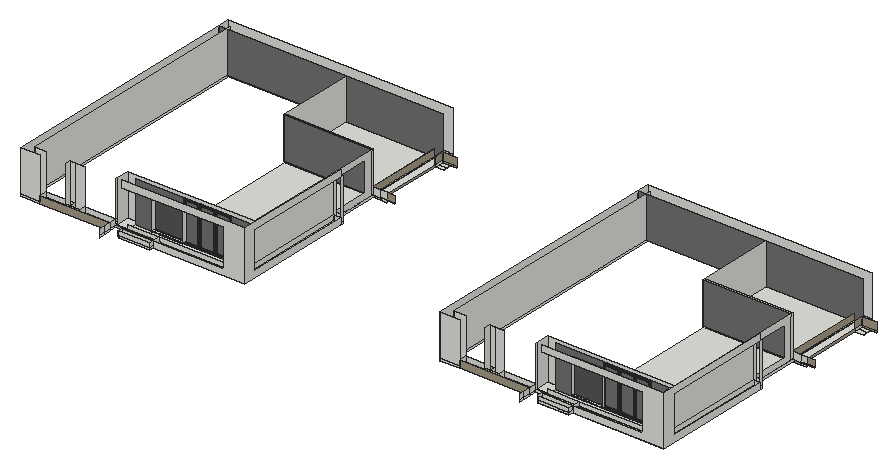
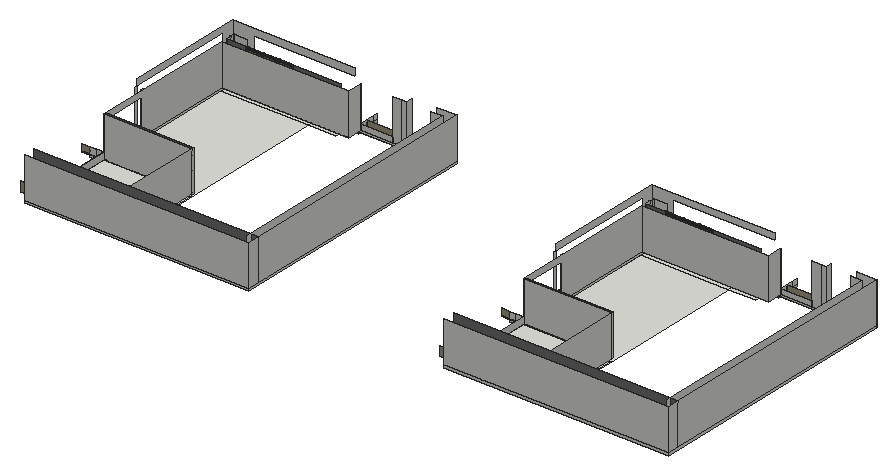
# SketchUp Ruby script. Lengths in inches.
U = 1.inch
M = Sketchup.active_model
def pt(a) = Geom::Point3d.new(a.map { |v| v * U })
def face(e, loops, mat)
  f = e.add_face(loops[0].map { |a| pt(a) })
  loops[1..].each { |l| e.add_face(l.map { |a| pt(a) }).erase! }
  f.material = f.back_material = mat if mat
  f
end
# faces: each face lists its corners as indices into pts; further lists are holes
def faces(e, pts, list, mat = nil) = list.each { |f| face(e, (f[0].is_a?(Array) ? f : [f]).map { |l| l.map { |i| pts[i] } }, mat) }
# xy, xz, yz: faces in a plane at the given z, y or x. An outline is a flat list of corners, or four numbers for a rectangle; further outlines are holes
def ring(l) = l.size == 4 ? [[l[0], l[1]], [l[2], l[1]], [l[2], l[3]], [l[0], l[3]]] : l.each_slice(2).to_a
def flat(e, list, mat, &to3) = list.each { |f| face(e, (f[0].is_a?(Array) ? f : [f]).map { |l| ring(l).map { |u, v| to3.(u, v) } }, mat) }
def xy(e, z, list, mat = nil) = flat(e, list, mat) { |x, y| [x, y, z] }
def xz(e, y, list, mat = nil) = flat(e, list, mat) { |x, z| [x, y, z] }
def yz(e, x, list, mat = nil) = flat(e, list, mat) { |y, z| [x, y, z] }
def lines(e, pts, list) = list.each { |a, b| e.add_line(pt(pts[a]), pt(pts[b])) }
# prism: a flat outline (further loops are holes) pulled along v
def prism(e, loops, v, mat = nil)
  f = face(e, loops, mat); d = Geom::Vector3d.new(v.map { |x| x * U })
  f.pushpull(f.normal.samedirection?(d) ? d.length : -d.length)
end
def box(e, o, s, mat = nil) = prism(e, [[o, [o[0] + s[0], o[1], o[2]], [o[0] + s[0], o[1] + s[1], o[2]], [o[0], o[1] + s[1], o[2]]]], [0, 0, s[2]], mat)
def at(x, y, z, deg = 0) = Geom::Transformation.translation(pt([x, y, z])) * Geom::Transformation.rotation(ORIGIN, Z_AXIS, deg.degrees)
def axes(o, x, y, z) = Geom::Transformation.new([*x, 0, *y, 0, *z, 0, *pt(o).to_a, 1])
def part(name) = M.definitions.add(name)
# library, detail: a bought-in or finely detailed component or shape, given as its bounding box
def library(name, o, s) = part(name).tap { |d| box(d.entities, o, s) }
def detail(e, o, s) = box(e.add_group.entities, o, s)
def put(e, d, t, mat = nil) = e.add_instance(d, t).tap { |i| i.material = mat if mat }
def group(e, t, mat = nil) = e.add_group.tap { |g| g.transformation = t; g.material = mat if mat }.entities
root = M.entities
M.materials.add("Wine2").color = [0, 0, 0]
M.materials["Wine2"].alpha = 0
M.materials.add("[0130_Gainsboro]").color = [39, 45, 50]
M.materials.add("[Color M05]").color = [114, 114, 114]
M.materials.add("[Color M06]").color = [86, 86, 86]
M.materials.add("[Concrete Tile]").color = [165, 155, 133]
M.materials.add("[Granite Brown]").color = [89, 59, 61]
c1 = part("Framed glazing panel")
xy(c1.entities,0,[[0,-0.98,43.07,0],[0,0,43.07,1.4]],"[0130_Gainsboro]")
xy(c1.entities,0.3,[[0.3,-1.43,42.77,-0.98]],"[0130_Gainsboro]")
xy(c1.entities,2.95,[[2.95,-1.43,40.12,-0.63],[2.95,-0.63,40.12,0],[2.95,0,40.12,0.64],[2.95,0.64,40.12,1.4]],"[0130_Gainsboro]")
xy(c1.entities,3.54,[[3.54,-0.63,39.53,0],[3.54,0,39.53,0.64]],"[0130_Gainsboro]")
xy(c1.entities,111.8125,[[3.54,-0.63,39.53,0],[3.54,0,39.53,0.64]],"[0130_Gainsboro]")
xy(c1.entities,112.4,[[2.95,-1.43,40.12,-0.63],[2.95,-0.63,40.12,0],[2.95,0,40.12,0.64],[2.95,0.64,40.12,1.4]],"[0130_Gainsboro]")
xy(c1.entities,115.05,[[0.3,-1.43,42.77,-0.98]],"[0130_Gainsboro]")
xy(c1.entities,115.35,[[0,-0.98,43.07,0],[0,0,43.07,1.4]],"[0130_Gainsboro]")
xz(c1.entities,-1.43,[[[0.3,0.3,42.77,115.05],[2.95,2.95,40.12,112.4]]],"[0130_Gainsboro]")
xz(c1.entities,-0.98,[[[0,0,43.07,115.35],[0.3,0.3,42.77,115.05]]],"[0130_Gainsboro]")
xz(c1.entities,-0.63,[[[2.95,2.95,40.12,112.4],[3.54,3.54,39.53,111.8125]]],"[0130_Gainsboro]")
xz(c1.entities,0,[[3.54,3.54,39.53,111.8125]],"Wine2")
xz(c1.entities,0,[[[0,0,43.07,115.35],[2.95,2.95,40.12,112.4]],[[2.95,2.95,40.12,112.4],[3.54,3.54,39.53,111.8125]]],"[0130_Gainsboro]")
xz(c1.entities,0.64,[[[2.95,2.95,40.12,112.4],[3.54,3.54,39.53,111.8125]]],"[0130_Gainsboro]")
xz(c1.entities,1.4,[[[0,0,43.07,115.35],[2.95,2.95,40.12,112.4]]],"[0130_Gainsboro]")
yz(c1.entities,0,[[-0.98,0,0,115.35],[0,0,1.4,115.35]],"[0130_Gainsboro]")
yz(c1.entities,0.3,[[-1.43,0.3,-0.98,115.05]],"[0130_Gainsboro]")
yz(c1.entities,2.95,[[-1.43,2.95,-0.63,112.4],[-0.63,2.95,0,112.4],[0,2.95,0.64,112.4],[0.64,2.95,1.4,112.4]],"[0130_Gainsboro]")
yz(c1.entities,3.54,[[-0.63,3.54,0,111.8125],[0,3.54,0.64,111.8125]],"[0130_Gainsboro]")
yz(c1.entities,39.53,[[-0.63,3.54,0,111.8125],[0,3.54,0.64,111.8125]],"[0130_Gainsboro]")
yz(c1.entities,40.12,[[-1.43,2.95,-0.63,112.4],[-0.63,2.95,0,112.4],[0,2.95,0.64,112.4],[0.64,2.95,1.4,112.4]],"[0130_Gainsboro]")
yz(c1.entities,42.77,[[-1.43,0.3,-0.98,115.05]],"[0130_Gainsboro]")
yz(c1.entities,43.07,[[-0.98,0,0,115.35],[0,0,1.4,115.35]],"[0130_Gainsboro]")
c2 = part("Glazed panel assembly")
put(c2.entities,c1,axes([90.57,1.43,0],[1.05148,0,0],[0,1,0],[0,0,1]))
put(c2.entities,c1,axes([0,1.43,0],[1.05148,0,0],[0,1,0],[0,0,1]))
put(c2.entities,c1,axes([45.29,1.43,0],[1.05148,0,0],[0,1,0],[0,0,1]))
xy(root,882,[[558.21,1786.97,648.68,1822.9375],[1776.4,1786.97,1866.87,1822.9375],[319.53,1799.9375,319.53,1822.9375,403.03,1822.9375,403.03,1806.5625,446.15,1806.5625,446.15,1822.9375,523.04,1822.9375,523.04,1799.9375],[648.68,1799.9375,648.68,1822.9375,890.875,1822.9375,890.875,1842.5,913.875,1842.5,913.875,1799.9375],[1537.72,1799.9375,1537.72,1822.9375,1621.22,1822.9375,1621.22,1806.5625,1664.33,1806.5625,1664.33,1822.9375,1741.23,1822.9375,1741.23,1799.9375],
  [1866.87,1799.9375,1866.87,1822.9375,2109.0625,1822.9375,2109.0625,1842.5,2132.0625,1842.5,2132.0625,1799.9375],[431.33,1806.5625,446.15,1822.9375],[1649.52,1806.5625,1664.33,1822.9375],[523.04,1822.9375,557.4,1822.9375,557.4,1826.625,557.88,1826.625,557.88,1830.25,523.04,1830.25],[648.68,1822.9375,890.875,1822.9375,890.875,1842.5,635.3125,1842.5,635.3125,1826.625,648.68,1826.625],
  [1741.23,1822.9375,1775.59,1822.9375,1775.59,1826.625,1776.07,1826.625,1776.07,1830.25,1741.23,1830.25],[1866.87,1822.9375,2109.0625,1822.9375,2109.0625,1842.5,1853.5,1842.5,1853.5,1826.625,1866.87,1826.625],[557.88,1826.625,635.3125,1830.25],[1776.07,1826.625,1853.5,1830.25],[557.88,1830.25,635.3125,1842.5],
  [1776.07,1830.25,1853.5,1842.5],[557.4,1842.5,635.3125,1869.5],[635.3125,1842.5,890.875,1869.5],[890.875,1842.5,891.6875,1869.5],[891.6875,1842.5,894.3125,2148.83],
  [894.3125,1842.5,913.875,2148.83],[1775.59,1842.5,1853.5,1869.5],[1853.5,1842.5,2109.0625,1869.5],[2109.0625,1842.5,2109.875,1869.5],[2109.875,1842.5,2112.5,2148.83],
  [2112.5,1842.5,2132.0625,2148.83],[635.3125,1869.5,890.875,2295.875],[1853.5,1869.5,2109.0625,2295.875],[894,2148.83,894.3125,2156.01],[894.3125,2148.83,913.875,2156.01],
  [2112.1875,2148.83,2112.5,2156.01],[2112.5,2148.83,2132.0625,2156.01],[635.3125,2295.875,637.0625,2518.89],[637.0625,2295.875,637.0625,2518.89,889.625,2518.89,889.625,2492.875,890.875,2492.875,890.875,2295.875],[1853.5,2295.875,1855.25,2518.89],
  [1855.25,2295.875,1855.25,2518.89,2107.8125,2518.89,2107.8125,2492.875,2109.0625,2492.875,2109.0625,2295.875],[889.625,2492.875,890.875,2518.89],[890.875,2492.875,912.625,2505.5625],[912.625,2492.875,913.875,2505.5625],[913.875,2492.875,938.375,2505.5625],
  [938.375,2492.875,938.5625,2518.89],[2107.8125,2492.875,2109.0625,2518.89],[2109.0625,2492.875,2130.8125,2505.5625],[2130.8125,2492.875,2132.0625,2505.5625],[2132.0625,2492.875,2156.5625,2505.5625],
  [2156.5625,2492.875,2156.75,2518.89],[890.875,2505.5625,912.625,2518.89],[912.625,2505.5625,913.875,2518.89],[913.875,2505.5625,938.375,2518.89],[2109.0625,2505.5625,2130.8125,2518.89],
  [2130.8125,2505.5625,2132.0625,2518.89],[2132.0625,2505.5625,2156.5625,2518.89],[635.3125,2518.89,890.875,2531.375],[1853.5,2518.89,2109.0625,2531.375]])
xy(root,882,[[890.875,2295.875,913.875,2492.875],[2109.0625,2295.875,2132.0625,2492.875]],"[Concrete Tile]")
xy(root,882,[[557.4,1822.9375,557.88,1826.625],[1775.59,1822.9375,1776.07,1826.625]],"[Granite Brown]")
xy(root,888,[[557.88,1786.97,558.21,1799.9375],[558.21,1786.97,647.87,1799.9375],[647.87,1786.97,648.68,1799.9375],[1776.07,1786.97,1776.4,1799.9375],[1776.4,1786.97,1866.06,1799.9375],
  [1866.06,1786.97,1866.87,1799.9375],[557.88,1799.9375,558.21,1822.9375],[558.21,1799.9375,647.87,1822.9375],[647.87,1799.9375,648.68,1822.9375],[1776.07,1799.9375,1776.4,1822.9375],
  [1776.4,1799.9375,1866.06,1822.9375],[1866.06,1799.9375,1866.87,1822.9375],[523.04,1822.9375,557.4,1826.625],[648.68,1822.9375,890.875,1826.625],[1741.23,1822.9375,1775.59,1826.625],
  [1866.87,1822.9375,2109.0625,1826.625],[523.04,1826.625,523.04,1865.75,557.4,1865.75,557.4,1850.9375,557.88,1850.9375,557.88,1826.625],[557.88,1826.625,890.875,1850.9375],[1741.23,1826.625,1741.23,1865.75,1775.59,1865.75,1775.59,1850.9375,1776.07,1850.9375,1776.07,1826.625],[1776.07,1826.625,2109.0625,1850.9375],
  [557.4,1850.9375,890.875,1865.75],[1775.59,1850.9375,2109.0625,1865.75],[894.3125,2148.83,913.875,2156.01],[2112.5,2148.83,2132.0625,2156.01],[635.3125,2290,890.875,2295.875],
  [1853.5,2290,2109.0625,2295.875],[890.875,2295.875,890.875,2517.14,912.625,2517.14,912.625,2492.875,913.875,2492.875,913.875,2295.875],[2109.0625,2295.875,2109.0625,2517.14,2130.8125,2517.14,2130.8125,2492.875,2132.0625,2492.875,2132.0625,2295.875],[912.625,2492.875,913.875,2517.14],[2130.8125,2492.875,2132.0625,2517.14],
  [890.875,2517.14,912.625,2518.64],[912.625,2517.14,913.875,2518.64],[2109.0625,2517.14,2130.8125,2518.64],[2130.8125,2517.14,2132.0625,2518.64],[890.875,2518.64,912.625,2518.89],
  [912.625,2518.64,913.875,2518.89],[2109.0625,2518.64,2130.8125,2518.89],[2130.8125,2518.64,2132.0625,2518.89],[285.875,2519.125,890.875,2531.375],[1504.0625,2519.125,2109.0625,2531.375]])
xy(root,888,[[557.4,1786.97,557.88,1799.9375],[1775.59,1786.97,1776.07,1799.9375],[557.4,1822.9375,557.88,1826.625],[1775.59,1822.9375,1776.07,1826.625]],"[Granite Brown]")
xy(root,889.75,[[635.3125,2295.875,889.625,2517.14],[889.625,2295.875,890.875,2517.14],[1853.5,2295.875,2107.8125,2517.14],[2107.8125,2295.875,2109.0625,2517.14]])
xy(root,895.375,[[632.49,1842.5,648.79,1850.9375],[648.79,1842.5,650.48,1850.9375],[650.48,1842.5,701.59,1850.9375],[1850.67,1842.5,1866.98,1850.9375],[1866.98,1842.5,1868.66,1850.9375],
  [1868.66,1842.5,1919.77,1850.9375]])
xy(root,895.6875,[[611.65,1842.5,632.49,1850.9375],[1829.84,1842.5,1850.67,1850.9375]])
xz(root,1786.97,[[558.21,882,648.68,888],[1776.4,882,1866.87,888],[557.88,888,647.87,900.6875],[1776.07,888,1866.06,900.6875]])
xz(root,1786.97,[[557.4,888,557.88,900.6875],[1775.59,888,1776.07,900.6875]],"[Granite Brown]")
xz(root,1799.9375,[[262.875,882,319.53,888],[648.68,882,913.875,882,913.875,1026.6875,557.88,1026.6875,557.88,1008,852.99,1008,852.99,900.6875,647.87,900.6875,647.87,888,648.68,888],[1481.0625,882,1537.72,888],[1866.87,882,2132.0625,882,2132.0625,1026.6875,1776.07,1026.6875,1776.07,1008,2071.18,1008,2071.18,900.6875,1866.06,900.6875,1866.06,888,1866.87,888],[262.875,888,319.53,1008],
  [557.4,888,647.87,900.6875],[1481.0625,888,1537.72,1008],[1775.59,888,1866.06,900.6875]])
xz(root,1799.9375,[[319.53,882,523.04,903.4375],[1537.72,882,1741.23,903.4375]],"[Concrete Tile]")
xz(root,1806.5625,[[403.0625,888,403.0625,903.4375,388.33,903.51,388.25,888.07],[403.0625,888,403.14,903.4375,403.0625,903.4375],[403.0625,888,431.33,888,431.33,903.4375,403.14,903.4375],[1621.25,888,1621.25,903.4375,1606.52,903.51,1606.4375,888.07],[1621.25,888,1621.33,903.4375,1621.25,903.4375],
  [1621.25,888,1649.52,888,1649.52,903.4375,1621.33,903.4375]])
xz(root,1822.9375,[[285.875,882,557.4,888],[558.21,882,648.68,888],[648.68,882,890.875,888],[1504.0625,882,1775.59,888],[1776.4,882,1866.87,888],
  [1866.87,882,2109.0625,888],[285.875,888,319.53,1008],[319.53,888,403.0625,888,388.25,888.07,388.33,903.4375,319.53,903.4375],[403.0625,888,388.25,888.07,388.33,903.4375,403.0625,903.4375],[403.0625,888,403.66,1008,388.85,1008,388.33,903.4375,403.0625,903.4375],
  [403.0625,888,403.66,1008,431.33,1008,431.33,888],[431.33,888,523.04,903.4375],[557.88,888,647.87,900.6875],[647.87,888,647.87,900.6875,852.99,900.6875,852.99,1008,890.875,1008,890.875,888],[1504.0625,888,1537.72,1008],
  [1537.72,888,1621.25,888,1606.4375,888.07,1606.52,903.4375,1537.72,903.4375],[1621.25,888,1606.4375,888.07,1606.52,903.4375,1621.25,903.4375],[1621.25,888,1621.85,1008,1607.04,1008,1606.52,903.4375,1621.25,903.4375],[1621.25,888,1621.85,1008,1649.52,1008,1649.52,888],[1649.52,888,1741.23,903.4375],
  [1776.07,888,1866.06,900.6875],[1866.06,888,1866.06,900.6875,2071.18,900.6875,2071.18,1008,2109.0625,1008,2109.0625,888]])
xz(root,1822.9375,[[557.4,882,557.88,888],[1775.59,882,1776.07,888]],"[Granite Brown]")
xz(root,1826.625,[[557.4,882,648.68,888],[1775.59,882,1866.87,888]])
xz(root,1835.1875,[[890.875,888,894.3125,1008],[2109.0625,888,2112.5,1008]])
xz(root,1842.5,[[632.49,893.4375,701.59,893.4375,701.59,895.375,632.49,895.375,632.49,895.6875,611.65,895.6875,611.65,893.75,632.49,893.75],[1850.67,893.4375,1919.77,893.4375,1919.77,895.375,1850.67,895.375,1850.67,895.6875,1829.84,895.6875,1829.84,893.75,1850.67,893.75]])
xz(root,1850.9375,[[[557.88,888,890.875,888,890.875,1008,557.88,1008,557.88,986.96,557.4,986.96,557.4,934.68,557.88,934.68],[632.49,895.375,632.49,895.6875,611.65,895.6875,611.65,991.5625,701.59,991.5625,701.59,895.375]],[[1776.07,888,2109.0625,888,2109.0625,1008,1776.07,1008,1776.07,986.96,1775.59,986.96,1775.59,934.68,1776.07,934.68],[1850.67,895.375,1850.67,895.6875,1829.84,895.6875,1829.84,991.5625,1919.77,991.5625,1919.77,895.375]]],"[Color M05]")
xz(root,1850.9375,[[632.49,895.375,701.59,895.375,701.59,991.5625,611.65,991.5625,611.65,895.6875,632.49,895.6875],[1850.67,895.375,1919.77,895.375,1919.77,991.5625,1829.84,991.5625,1829.84,895.6875,1850.67,895.6875]],"[Color M06]")
xz(root,1865.75,[[523.04,888,890.875,1008],[1741.23,888,2109.0625,1008]])
xz(root,2148.83,[[894.3125,882,913.875,888],[2112.5,882,2132.0625,888],[894.3125,888,913.875,900.6875],[2112.5,888,2132.0625,900.6875]])
xz(root,2156.01,[[894.3125,882,913.875,888],[2112.5,882,2132.0625,888],[894.3125,888,913.875,905.36],[2112.5,888,2132.0625,905.36]])
xz(root,2290,[[635.3125,888,890.875,1008],[1853.5,888,2109.0625,1008]],"[Color M05]")
xz(root,2295.875,[[913.875,882,930.75,888],[2132.0625,882,2148.9375,888],[635.3125,888,890.875,889.75],[890.875,888,913.875,908.8125],[913.875,888,930.75,889.75],
  [930.75,888,954.6875,889.75],[1853.5,888,2109.0625,889.75],[2109.0625,888,2132.0625,908.8125],[2132.0625,888,2148.9375,889.75],[2148.9375,888,2172.875,889.75],
  [635.3125,889.75,635.3125,1008,890.875,1008,890.875,908.8125,889.625,908.8125,889.625,889.75],[889.625,889.75,890.875,908.8125],[913.875,889.75,930.75,908.8125],[1853.5,889.75,1853.5,1008,2109.0625,1008,2109.0625,908.8125,2107.8125,908.8125,2107.8125,889.75],[2107.8125,889.75,2109.0625,908.8125],
  [2132.0625,889.75,2148.9375,908.8125]])
xz(root,2295.875,[[930.75,889.75,954.6875,908.8125],[2148.9375,889.75,2172.875,908.8125]],"[Concrete Tile]")
xz(root,2492.875,[[912.625,882,913.875,888],[2130.8125,882,2132.0625,888],[912.625,888,913.875,908.8125],[2130.8125,888,2132.0625,908.8125]])
xz(root,2517.14,[[889.625,889.75,890.875,908.8125],[2107.8125,889.75,2109.0625,908.8125]])
xz(root,2518.64,[[912.625,888,913.875,908.8125],[2130.8125,888,2132.0625,908.8125]])
xz(root,2518.89,[[912.625,882,913.875,888],[2130.8125,882,2132.0625,888]])
xz(root,2518.89,[[913.875,882,954.6875,908.8125],[2132.0625,882,2172.875,908.8125]],"[Concrete Tile]")
xz(root,2519.125,[[262.875,888,913.875,1008],[1481.0625,888,2132.0625,1008]],"[Color M05]")
xz(root,2531.375,[[285.875,882,890.875,888],[1504.0625,882,2109.0625,888]])
xz(root,2554.375,[[262.875,882,913.875,888],[1481.0625,882,2132.0625,888],[262.875,888,913.875,1008],[1481.0625,888,2132.0625,1008]])
yz(root,262.875,[[1799.9375,882,2554.375,888],[1799.9375,888,2519.125,1008],[2519.125,888,2554.375,1008]])
yz(root,285.875,[[1822.9375,882,2531.375,888],[1822.9375,888,2531.375,1008]])
yz(root,319.53,[[1799.9375,888,1822.9375,903.4375]])
yz(root,403.0625,[[1806.5625,888,1822.9375,903.4375]])
yz(root,431.33,[[1806.5625,888,1822.9375,903.4375]])
yz(root,523.04,[[1763.25,882,1799.9375,888],[1763.25,888,1799.9375,903.4375],[1799.9375,888,1822.9375,903.4375],[1822.9375,888,1826.625,1008],[1826.625,888,1865.75,1008]])
yz(root,557.4,[[1822.9375,882,1826.625,888],[1786.97,888,1799.9375,900.6875]])
yz(root,558.21,[[1786.97,882,1822.9375,888]])
yz(root,611.65,[[1842.5,895.6875,1850.9375,991.5625]])
yz(root,632.49,[[1842.5,895.375,1850.9375,895.6875]])
yz(root,635.3125,[[2290,888,2295.875,1008],[2295.875,889.75,2517.14,1008]])
yz(root,647.87,[[1786.97,888,1799.9375,900.6875],[1799.9375,888,1822.9375,900.6875]])
yz(root,648.68,[[1786.97,882,1799.9375,888],[1799.9375,882,1822.9375,888],[1822.9375,882,1826.625,888]])
yz(root,701.59,[[1842.5,895.375,1850.9375,991.5625]])
yz(root,889.625,[[2295.875,889.75,2517.14,908.8125]])
yz(root,890.875,[[1822.9375,882,2531.375,888],[1822.9375,888,1826.625,1008],[1826.625,888,1835.1875,1008],[1835.1875,888,1850.9375,1008],[[1865.75,888,2290,1008],[2156.01,905.36,2266.33,991.04]],
  [2290,888,2295.875,889.75],[2295.875,888,2517.14,889.75],[2517.14,888,2518.64,889.75],[2518.64,888,2518.89,889.75],[2290,889.75,2295.875,1008]])
yz(root,890.875,[[2295.875,889.75,2517.14,908.8125]],"[Concrete Tile]")
yz(root,894.3125,[[2148.83,882,2156.01,888],[1835.1875,888,2148.83,900.6875],[2148.83,888,2156.01,1008]])
yz(root,912.625,[[2492.875,882,2518.89,888],[2492.875,888,2518.64,908.8125]])
yz(root,913.875,[[1799.9375,882,2148.83,882,2148.83,900.6875,1835.1875,900.6875,1835.1875,1008,2148.83,1008,2148.83,1026.6875,1799.9375,1026.6875],[2148.83,882,2156.01,888],[2492.875,882,2518.89,888],[2518.89,882,2520.14,888],[2148.83,888,2156.01,1008],
  [2518.64,888,2518.89,908.8125],[2518.89,888,2519.125,908.8125],[2519.125,888,2520.14,908.8125]])
yz(root,913.875,[[2295.875,882,2492.875,888],[2492.875,888,2518.64,908.8125]],"[Concrete Tile]")
yz(root,1481.0625,[[1799.9375,882,2554.375,888],[1799.9375,888,2519.125,1008],[2519.125,888,2554.375,1008]])
yz(root,1504.0625,[[1822.9375,882,2531.375,888],[1822.9375,888,2531.375,1008]])
yz(root,1537.72,[[1799.9375,888,1822.9375,903.4375]])
yz(root,1621.25,[[1806.5625,888,1822.9375,903.4375]])
yz(root,1649.52,[[1806.5625,888,1822.9375,903.4375]])
yz(root,1741.23,[[1763.25,882,1799.9375,888],[1763.25,888,1799.9375,903.4375],[1799.9375,888,1822.9375,903.4375],[1822.9375,888,1826.625,1008],[1826.625,888,1865.75,1008]])
yz(root,1775.59,[[1822.9375,882,1826.625,888],[1786.97,888,1799.9375,900.6875]])
yz(root,1776.4,[[1786.97,882,1822.9375,888]])
yz(root,1829.84,[[1842.5,895.6875,1850.9375,991.5625]])
yz(root,1850.67,[[1842.5,895.375,1850.9375,895.6875]])
yz(root,1853.5,[[2290,888,2295.875,1008],[2295.875,889.75,2517.14,1008]])
yz(root,1866.06,[[1786.97,888,1799.9375,900.6875],[1799.9375,888,1822.9375,900.6875]])
yz(root,1866.87,[[1786.97,882,1799.9375,888],[1799.9375,882,1822.9375,888],[1822.9375,882,1826.625,888]])
yz(root,1919.77,[[1842.5,895.375,1850.9375,991.5625]])
yz(root,2107.8125,[[2295.875,889.75,2517.14,908.8125]])
yz(root,2109.0625,[[1822.9375,882,2531.375,888],[1822.9375,888,1826.625,1008],[1826.625,888,1835.1875,1008],[1835.1875,888,1850.9375,1008],[[1865.75,888,2290,1008],[2156.01,905.36,2266.33,991.04]],
  [2290,888,2295.875,889.75],[2295.875,888,2517.14,889.75],[2517.14,888,2518.64,889.75],[2518.64,888,2518.89,889.75],[2290,889.75,2295.875,1008]])
yz(root,2109.0625,[[2295.875,889.75,2517.14,908.8125]],"[Concrete Tile]")
yz(root,2112.5,[[2148.83,882,2156.01,888],[1835.1875,888,2148.83,900.6875],[2148.83,888,2156.01,1008]])
yz(root,2130.8125,[[2492.875,882,2518.89,888],[2492.875,888,2518.64,908.8125]])
yz(root,2132.0625,[[1799.9375,882,2148.83,882,2148.83,900.6875,1835.1875,900.6875,1835.1875,1008,2148.83,1008,2148.83,1026.6875,1799.9375,1026.6875],[2148.83,882,2156.01,888],[2492.875,882,2518.89,888],[2518.89,882,2520.14,888],[2148.83,888,2156.01,1008],
  [2518.64,888,2518.89,908.8125],[2518.89,888,2519.125,908.8125],[2519.125,888,2520.14,908.8125]])
yz(root,2132.0625,[[2295.875,882,2492.875,888],[2492.875,888,2518.64,908.8125]],"[Concrete Tile]")
p = [[403.0625,1822.9375,888],[403.0625,1806.5625,888],[388.25,1806.5625,888.07],[388.25,1822.9375,888.07],[1621.25,1822.9375,888],[1621.25,1806.5625,888],
  [1606.4375,1806.5625,888.07],[1606.4375,1822.9375,888.07],[388.33,1806.5625,903.51],[388.85,1806.5625,1008.07],[388.85,1822.9375,1008.07],[388.85,1822.9375,1008],
  [388.33,1822.9375,903.4375],[1606.52,1806.5625,903.51],[1607.04,1806.5625,1008.07],[1607.04,1822.9375,1008.07],[1607.04,1822.9375,1008],[1606.52,1822.9375,903.4375],
  [2132.0625,2517.14,888],[2172.875,2517.14,888],[1741.23,1778.3125,888],[1741.23,1778.3125,903.4375],[1741.23,1778.3125,882],[913.875,2517.14,888],
  [954.6875,2517.14,888],[523.04,1778.3125,888],[523.04,1778.3125,903.4375],[523.04,1778.3125,882]]
faces(root,p,[[0,1,2,3],[4,5,6,7],[3,2,8,9,10,11,12],[7,6,13,14,15,16,17]])
lines(root,p,[[18,19],[20,21],[22,20],[23,24],[25,26],[27,25]])
put(root,c2,at(1916.05,1848.87,891.83))
put(root,c2,at(697.86,1848.87,891.83))
